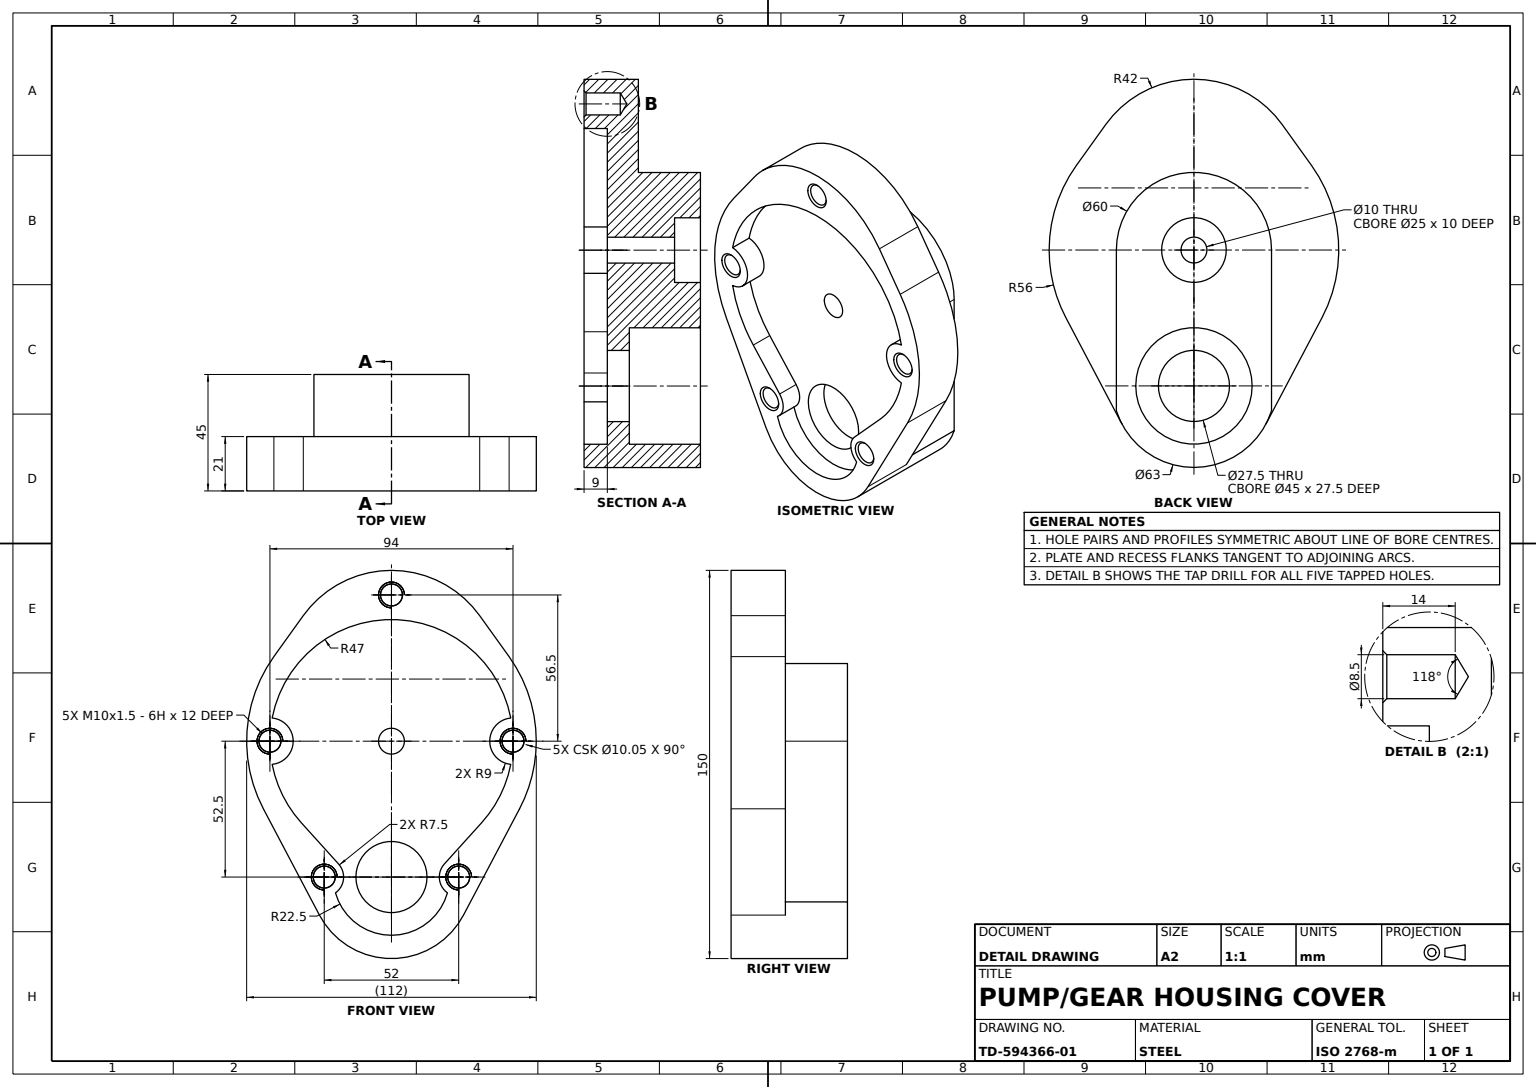
solid
v1 (0,48.5,34.11378)
v2 (21,48.5,34.11378)
e1 v1 v2 LINE
v3 (21,48.5,-34.11378)
e2 v3 v2 CIRCLE(AX(P(21,24,0),D(1,0,0),D(0,0,-1)),42)
v4 (0,48.5,-34.11378)
e3 v4 v3 LINE
e4 v4 v1 CIRCLE(AX(P(0,24,0),D(1,0,0),D(0,0,-1)),42)
face CYL(AX(P(0,24,0),D(1,0,0),D(0,0,-1)),42) [e1 -e2 -e3 e4]
v5 (20.225,0,42.75)
v6 (21,0,41.975)
e5 v5 v6 LINE
v7 (20.225,0,51.25)
e6 v7 v5 CIRCLE(AX(P(20.225,0,47),D(1,0,0),D(0,0,-1)),4.25)
v8 (21,0,52.025)
e7 v7 v8 LINE
e8 v8 v6 CIRCLE(AX(P(21,0,47),D(1,0,0),D(0,0,-1)),5.025)
face CONE(AX(P(21,0,47),D(1,0,0),D(0,0,-1)),5.025,0.785398163) rev [-e5 -e6 e7 e8]
v9 (12,-31.528256,-34.856407)
v10 (21,-31.528256,-34.856407)
e9 v9 v10 LINE
v11 (12,-47.468895,-20.437807)
e10 v11 v9 LINE
v12 (21,-47.468895,-20.437807)
e11 v11 v12 LINE
e12 v12 v10 LINE
face PLANE(AX(P(12,-47.468895,-20.437807),D(0,-0.670813951,-0.741625676),D(0,0.741625676,-0.670813951))) rev [-e9 -e10 e11 e12]
v13 (7,-52.5,30.25)
v14 (7,-52.5,21.75)
e13 v13 v14 CIRCLE(AX(P(7,-52.5,26),D(1,0,0),D(0,0,-1)),4.25)
v15 (4.446342,-52.5,26)
e14 v15 v14 LINE
e15 v15 v13 LINE
face CONE(AX(P(7,-52.5,26),D(1,0,0),D(0,0,-1)),4.25,1.029744259) rev [e13 -e14 e15]
v16 (12,-52.5,13.75)
v17 (3.5,-52.5,13.75)
e16 v16 v17 LINE
v18 (12,-52.5,-13.75)
e17 v16 v18 CIRCLE(AX(P(12,-52.5,0),D(1,0,0),D(0,0,-1)),13.75)
v19 (3.5,-52.5,-13.75)
e18 v18 v19 LINE
e19 v19 v17 CIRCLE(AX(P(3.5,-52.5,0),D(-1,0,0),D(0,0,1)),13.75)
face CYL(AX(P(-24,-52.5,0),D(-1,0,0),D(0,0,1)),13.75) rev [-e16 e17 e18 e19]
v20 (7,0,42.75)
v21 (7,0,51.25)
e20 v20 v21 CIRCLE(AX(P(7,0,47),D(1,0,0),D(0,0,-1)),4.25)
v22 (4.446342,0,47)
e21 v22 v21 LINE
e22 v22 v20 LINE
face CONE(AX(P(7,0,47),D(1,0,0),D(0,0,-1)),4.25,1.029744259) rev [e20 -e21 e22]
v23 (12,-47.468895,20.437807)
v24 (21,-47.468895,20.437807)
e23 v23 v24 LINE
v25 (12,-31.528256,34.856407)
e24 v25 v23 LINE
v26 (21,-31.528256,34.856407)
e25 v25 v26 LINE
e26 v26 v24 LINE
face PLANE(AX(P(12,-47.468895,20.437807),D(0,-0.670813951,0.741625676),D(0,-0.741625676,-0.670813951))) rev [-e23 -e24 e25 e26]
v27 (-24,0,12.5)
v28 (-24,0,-12.5)
e27 v27 v28 CIRCLE(AX(P(-24,0,0),D(-1,0,0),D(0,0,1)),12.5)
v29 (-14,0,-12.5)
e28 v29 v28 LINE
v30 (-14,0,12.5)
e29 v30 v29 CIRCLE(AX(P(-14,0,0),D(-1,0,0),D(0,0,1)),12.5)
e30 v30 v27 LINE
face CYL(AX(P(-24,0,0),D(-1,0,0),D(0,0,1)),12.5) rev [e27 -e28 -e29 e30]
v31 (0,32.666667,45.48504)
e31 v1 v31 LINE
v32 (21,32.666667,45.48504)
e32 v31 v32 LINE
e33 v2 v32 LINE
face PLANE(AX(P(0,32.666667,45.48504),D(0,0.583333333,0.812232862),D(0,-0.812232862,0.583333333))) [-e1 e31 e32 -e33]
v33 (-24,-62.104686,-30)
v34 (0,-62.104686,-30)
e34 v33 v34 LINE
v35 (-24,0,-30)
e35 v35 v33 LINE
v36 (0,0,-30)
e36 v35 v36 LINE
e37 v36 v34 LINE
face PLANE(AX(P(-24,0,-30),D(0,0,1),D(0,-1,0))) rev [-e34 -e35 e36 e37]
v37 (4.446342,0,-47)
v38 (7,0,-51.25)
e38 v37 v38 LINE
v39 (7,0,-42.75)
e39 v37 v39 LINE
e40 v39 v38 CIRCLE(AX(P(7,0,-47),D(1,0,0),D(0,0,-1)),4.25)
face CONE(AX(P(7,0,-47),D(1,0,0),D(0,0,-1)),4.25,1.029744259) rev [-e38 e39 e40]
v40 (0,-26.133333,-49.528264)
v41 (0,0,-56)
e41 v40 v41 CIRCLE(AX(P(0,0,0),D(1,0,0),D(0,0,-1)),56)
v42 (21,0,-56)
e42 v41 v42 LINE
v43 (21,-26.133333,-49.528264)
e43 v43 v42 CIRCLE(AX(P(21,0,0),D(1,0,0),D(0,0,-1)),56)
e44 v40 v43 LINE
face CYL(AX(P(0,0,0),D(1,0,0),D(0,0,-1)),56) [e41 e42 -e43 -e44]
v44 (20.225,-52.5,-21.75)
v45 (21,-52.5,-20.975)
e45 v44 v45 LINE
v46 (20.225,-52.5,-30.25)
e46 v46 v44 CIRCLE(AX(P(20.225,-52.5,-26),D(1,0,0),D(0,0,-1)),4.25)
v47 (21,-52.5,-31.025)
e47 v46 v47 LINE
e48 v47 v45 CIRCLE(AX(P(21,-52.5,-26),D(1,0,0),D(0,0,-1)),5.025)
face CONE(AX(P(21,-52.5,-26),D(1,0,0),D(0,0,-1)),5.025,0.785398163) rev [-e45 -e46 e47 e48]
e49 v21 v20 CIRCLE(AX(P(7,0,47),D(1,0,0),D(0,0,-1)),4.25)
face CONE(AX(P(7,0,47),D(1,0,0),D(0,0,-1)),4.25,1.029744259) rev [e21 e49 -e22]
v48 (20.225,-52.5,30.25)
e50 v13 v48 LINE
e51 v14 v13 CIRCLE(AX(P(7,-52.5,26),D(1,0,0),D(0,0,-1)),4.25)
v49 (20.225,-52.5,21.75)
e52 v14 v49 LINE
e53 v49 v48 CIRCLE(AX(P(20.225,-52.5,26),D(1,0,0),D(0,0,-1)),4.25)
face CYL(AX(P(21,-52.5,26),D(1,0,0),D(0,0,-1)),4.25) rev [-e50 -e51 e52 e53]
v50 (7,56.5,-4.25)
v51 (20.225,56.5,-4.25)
e54 v50 v51 LINE
v52 (20.225,56.5,4.25)
e55 v51 v52 CIRCLE(AX(P(20.225,56.5,0),D(1,0,0),D(0,0,-1)),4.25)
v53 (7,56.5,4.25)
e56 v53 v52 LINE
e57 v50 v53 CIRCLE(AX(P(7,56.5,0),D(1,0,0),D(0,0,-1)),4.25)
face CYL(AX(P(21,56.5,0),D(1,0,0),D(0,0,-1)),4.25) rev [e54 e55 -e56 -e57]
v54 (21,-26.133333,49.528264)
v55 (21,-67.2,27.859648)
e58 v54 v55 LINE
v56 (0,-26.133333,49.528264)
e59 v56 v54 LINE
v57 (0,-67.2,27.859648)
e60 v56 v57 LINE
e61 v57 v55 LINE
face PLANE(AX(P(0,-26.133333,49.528264),D(0,-0.466666667,0.884433277),D(0,-0.884433277,-0.466666667))) [-e58 -e59 e60 e61]
v58 (4.446342,56.5,0)
e62 v58 v53 LINE
e63 v58 v50 LINE
face CONE(AX(P(7,56.5,0),D(1,0,0),D(0,0,-1)),4.25,1.029744259) rev [-e62 e63 e57]
v59 (4.446342,-52.5,-26)
v60 (7,-52.5,-30.25)
e64 v59 v60 LINE
v61 (7,-52.5,-21.75)
e65 v60 v61 CIRCLE(AX(P(7,-52.5,-26),D(1,0,0),D(0,0,-1)),4.25)
e66 v59 v61 LINE
face CONE(AX(P(7,-52.5,-26),D(1,0,0),D(0,0,-1)),4.25,1.029744259) rev [e64 e65 -e66]
v62 (12,-8.958653,-46.138298)
v63 (21,-8.958653,-46.138298)
e67 v62 v63 LINE
v64 (21,8.958653,-46.138298)
e68 v63 v64 CIRCLE(AX(P(21,0,-47),D(-1,0,0),D(0,0,1)),9)
v65 (12,8.958653,-46.138298)
e69 v65 v64 LINE
e70 v62 v65 CIRCLE(AX(P(12,0,-47),D(-1,0,0),D(0,0,1)),9)
face CYL(AX(P(12,0,-47),D(1,0,0),D(0,0,-1)),9) [e67 e68 -e69 -e70]
v66 (12,8.958653,46.138298)
v67 (12,0,38)
e71 v66 v67 CIRCLE(AX(P(12,0,47),D(-1,0,0),D(0,0,-1)),9)
v68 (12,-8.958653,46.138298)
e72 v67 v68 CIRCLE(AX(P(12,0,47),D(-1,0,0),D(0,0,-1)),9)
e73 v68 v25 CIRCLE(AX(P(12,0,0),D(1,0,0),D(0,0,-1)),47)
v69 (12,-52.5,18.5)
e74 v23 v69 CIRCLE(AX(P(12,-52.5,26),D(-1,0,0),D(0,0,1)),7.5)
v70 (12,-58.61236,21.653846)
e75 v69 v70 CIRCLE(AX(P(12,-52.5,26),D(-1,0,0),D(0,0,1)),7.5)
v71 (12,-58.61236,-21.653846)
e76 v70 v71 CIRCLE(AX(P(12,-52.5,0),D(1,0,0),D(0,0,-1)),22.5)
e77 v71 v11 CIRCLE(AX(P(12,-52.5,-26),D(-1,0,0),D(0,0,-1)),7.5)
e78 v9 v62 CIRCLE(AX(P(12,0,0),D(1,0,0),D(0,0,-1)),47)
e79 v65 v66 CIRCLE(AX(P(12,0,0),D(1,0,0),D(0,0,-1)),47)
e80 v18 v16 CIRCLE(AX(P(12,-52.5,0),D(1,0,0),D(0,0,-1)),13.75)
v72 (12,0,5)
v73 (12,0,-5)
e81 v72 v73 CIRCLE(AX(P(12,0,0),D(1,0,0),D(0,0,-1)),5)
e82 v73 v72 CIRCLE(AX(P(12,0,0),D(1,0,0),D(0,0,-1)),5)
face PLANE(AX(P(12,0,0),D(1,0,0),D(0,0,-1))) [e71 e72 e73 e24 e74 e75 e76 e77 e10 e78 e70 e79] [-e17 -e80] [-e81 -e82]
e83 v48 v49 CIRCLE(AX(P(20.225,-52.5,26),D(1,0,0),D(0,0,-1)),4.25)
face CYL(AX(P(21,-52.5,26),D(1,0,0),D(0,0,-1)),4.25) rev [e50 e83 -e52 -e13]
v74 (-24,-62.104686,30)
v75 (-24,0,30)
e84 v74 v75 LINE
v76 (0,-62.104686,30)
e85 v74 v76 LINE
v77 (0,0,30)
e86 v76 v77 LINE
e87 v75 v77 LINE
face PLANE(AX(P(-24,0,30),D(0,0,-1),D(0,1,0))) rev [-e84 e85 e86 -e87]
e88 v17 v19 CIRCLE(AX(P(3.5,-52.5,0),D(-1,0,0),D(0,0,1)),13.75)
face CYL(AX(P(-24,-52.5,0),D(-1,0,0),D(0,0,1)),13.75) rev [e16 e88 -e18 e80]
v78 (21,56.5,-5.025)
e89 v51 v78 LINE
v79 (21,56.5,5.025)
e90 v78 v79 CIRCLE(AX(P(21,56.5,0),D(1,0,0),D(0,0,-1)),5.025)
e91 v52 v79 LINE
face CONE(AX(P(21,56.5,0),D(1,0,0),D(0,0,-1)),5.025,0.785398163) rev [e89 e90 -e91 -e55]
v80 (21,8.958653,46.138298)
e92 v64 v80 CIRCLE(AX(P(21,0,0),D(1,0,0),D(0,0,-1)),47)
e93 v66 v80 LINE
face CYL(AX(P(12,0,0),D(1,0,0),D(0,0,-1)),47) rev [-e79 e69 e92 -e93]
e94 v61 v60 CIRCLE(AX(P(7,-52.5,-26),D(1,0,0),D(0,0,-1)),4.25)
e95 v61 v44 LINE
e96 v44 v46 CIRCLE(AX(P(20.225,-52.5,-26),D(1,0,0),D(0,0,-1)),4.25)
e97 v60 v46 LINE
face CYL(AX(P(21,-52.5,-26),D(1,0,0),D(0,0,-1)),4.25) rev [-e94 e95 e96 -e97]
e98 v38 v39 CIRCLE(AX(P(7,0,-47),D(1,0,0),D(0,0,-1)),4.25)
face CONE(AX(P(7,0,-47),D(1,0,0),D(0,0,-1)),4.25,1.029744259) rev [e98 -e39 e38]
face CONE(AX(P(7,-52.5,26),D(1,0,0),D(0,0,-1)),4.25,1.029744259) rev [e51 -e15 e14]
face CONE(AX(P(7,-52.5,-26),D(1,0,0),D(0,0,-1)),4.25,1.029744259) rev [e94 -e64 e66]
v81 (21,-52.5,20.975)
e99 v49 v81 LINE
v82 (21,-52.5,31.025)
e100 v81 v82 CIRCLE(AX(P(21,-52.5,26),D(1,0,0),D(0,0,-1)),5.025)
e101 v48 v82 LINE
face CONE(AX(P(21,-52.5,26),D(1,0,0),D(0,0,-1)),5.025,0.785398163) rev [-e53 e99 e100 -e101]
face CYL(AX(P(21,-52.5,-26),D(1,0,0),D(0,0,-1)),4.25) rev [e97 e46 -e95 -e65]
v83 (-24,-52.5,-22.5)
v84 (-24,-52.5,22.5)
e102 v83 v84 CIRCLE(AX(P(-24,-52.5,0),D(-1,0,0),D(0,0,1)),22.5)
v85 (3.5,-52.5,22.5)
e103 v85 v84 LINE
v86 (3.5,-52.5,-22.5)
e104 v86 v85 CIRCLE(AX(P(3.5,-52.5,0),D(-1,0,0),D(0,0,1)),22.5)
e105 v86 v83 LINE
face CYL(AX(P(-24,-52.5,0),D(-1,0,0),D(0,0,1)),22.5) rev [e102 -e103 -e104 e105]
e106 v82 v81 CIRCLE(AX(P(21,-52.5,26),D(1,0,0),D(0,0,-1)),5.025)
face CONE(AX(P(21,-52.5,26),D(1,0,0),D(0,0,-1)),5.025,0.785398163) rev [-e83 e101 e106 -e99]
v87 (-14,0,5)
v88 (-14,0,-5)
e107 v87 v88 CIRCLE(AX(P(-14,0,0),D(-1,0,0),D(0,0,1)),5)
e108 v73 v88 LINE
e109 v72 v87 LINE
face CYL(AX(P(-24,0,0),D(-1,0,0),D(0,0,1)),5) rev [e107 -e108 e82 e109]
e110 v21 v7 LINE
e111 v20 v5 LINE
face CYL(AX(P(21,0,47),D(1,0,0),D(0,0,-1)),4.25) rev [-e49 e110 e6 -e111]
e112 v88 v87 CIRCLE(AX(P(-14,0,0),D(-1,0,0),D(0,0,1)),5)
face CYL(AX(P(-24,0,0),D(-1,0,0),D(0,0,1)),5) rev [e81 e108 e112 -e109]
v89 (21,0,38)
v90 (21,-8.958653,46.138298)
e113 v89 v90 CIRCLE(AX(P(21,0,47),D(-1,0,0),D(0,0,-1)),9)
e114 v68 v90 LINE
e115 v67 v89 LINE
face CYL(AX(P(12,0,47),D(1,0,0),D(0,0,-1)),9) [e113 -e114 -e72 e115]
v91 (21,0,-41.975)
v92 (21,0,-52.025)
e116 v91 v92 CIRCLE(AX(P(21,0,-47),D(1,0,0),D(0,0,-1)),5.025)
e117 v92 v91 CIRCLE(AX(P(21,0,-47),D(1,0,0),D(0,0,-1)),5.025)
v93 (21,-67.2,-27.859648)
e118 v93 v43 LINE
v94 (21,32.666667,-45.48504)
e119 v42 v94 CIRCLE(AX(P(21,0,0),D(1,0,0),D(0,0,-1)),56)
e120 v94 v3 LINE
e121 v32 v54 CIRCLE(AX(P(21,0,0),D(1,0,0),D(0,0,-1)),56)
e122 v55 v93 CIRCLE(AX(P(21,-52.5,0),D(1,0,0),D(0,0,-1)),31.5)
e123 v45 v47 CIRCLE(AX(P(21,-52.5,-26),D(1,0,0),D(0,0,-1)),5.025)
e124 v79 v78 CIRCLE(AX(P(21,56.5,0),D(1,0,0),D(0,0,-1)),5.025)
e125 v80 v89 CIRCLE(AX(P(21,0,47),D(-1,0,0),D(0,0,-1)),9)
e126 v10 v63 CIRCLE(AX(P(21,0,0),D(1,0,0),D(0,0,-1)),47)
v95 (21,-58.61236,-21.653846)
e127 v95 v12 CIRCLE(AX(P(21,-52.5,-26),D(-1,0,0),D(0,0,-1)),7.5)
v96 (21,-58.61236,21.653846)
e128 v96 v95 CIRCLE(AX(P(21,-52.5,0),D(1,0,0),D(0,0,-1)),22.5)
v97 (21,-52.5,18.5)
e129 v97 v96 CIRCLE(AX(P(21,-52.5,26),D(-1,0,0),D(0,0,1)),7.5)
e130 v24 v97 CIRCLE(AX(P(21,-52.5,26),D(-1,0,0),D(0,0,1)),7.5)
e131 v90 v26 CIRCLE(AX(P(21,0,0),D(1,0,0),D(0,0,-1)),47)
e132 v6 v8 CIRCLE(AX(P(21,0,47),D(1,0,0),D(0,0,-1)),5.025)
face PLANE(AX(P(21,0,0),D(1,0,0),D(0,0,-1))) [-e116 -e117] [e118 e43 e119 e120 e2 e33 e121 e58 e122] [-e48 -e123] [-e106 -e100] [-e124 -e90] [-e125 -e92 -e68 -e126 -e12 -e127 -e128 -e129 -e130 -e26 -e131 -e113] [-e8 -e132]
e133 v70 v96 LINE
e134 v71 v95 LINE
face CYL(AX(P(12,-52.5,0),D(1,0,0),D(0,0,-1)),22.5) rev [e133 e128 -e134 -e76]
face CONE(AX(P(21,-52.5,-26),D(1,0,0),D(0,0,-1)),5.025,0.785398163) rev [-e47 -e96 e45 e123]
e135 v69 v97 LINE
face CYL(AX(P(12,-52.5,26),D(1,0,0),D(0,0,-1)),7.5) [e130 -e135 -e74 e23]
e136 v29 v30 CIRCLE(AX(P(-14,0,0),D(-1,0,0),D(0,0,1)),12.5)
face PLANE(AX(P(-14,5,0),D(1,0,0),D(0,0,-1))) rev [e136 e29] [-e112 -e107]
face CYL(AX(P(12,-52.5,-26),D(1,0,0),D(0,0,-1)),7.5) [e127 -e11 -e77 e134]
e137 v53 v50 CIRCLE(AX(P(7,56.5,0),D(1,0,0),D(0,0,-1)),4.25)
face CONE(AX(P(7,56.5,0),D(1,0,0),D(0,0,-1)),4.25,1.029744259) rev [-e63 e62 e137]
v98 (0,32.666667,-45.48504)
e138 v41 v98 CIRCLE(AX(P(0,0,0),D(1,0,0),D(0,0,-1)),56)
e139 v98 v94 LINE
face CYL(AX(P(0,0,0),D(1,0,0),D(0,0,-1)),56) [-e119 -e42 e138 e139]
face CYL(AX(P(12,0,47),D(1,0,0),D(0,0,-1)),9) [-e115 -e71 e93 e125]
face CYL(AX(P(12,0,0),D(1,0,0),D(0,0,-1)),47) rev [e9 e126 -e67 -e78]
e140 v98 v4 LINE
face PLANE(AX(P(0,32.666667,-45.48504),D(0,0.583333333,-0.812232862),D(0,0.812232862,0.583333333))) [-e120 -e139 e140 e3]
e141 v31 v56 CIRCLE(AX(P(0,0,0),D(1,0,0),D(0,0,-1)),56)
face CYL(AX(P(0,0,0),D(1,0,0),D(0,0,-1)),56) [-e121 -e32 e141 e59]
v99 (20.225,0,-42.75)
v100 (20.225,0,-51.25)
e142 v99 v100 CIRCLE(AX(P(20.225,0,-47),D(1,0,0),D(0,0,-1)),4.25)
e143 v38 v100 LINE
e144 v39 v99 LINE
face CYL(AX(P(21,0,-47),D(1,0,0),D(0,0,-1)),4.25) rev [e142 -e143 -e40 e144]
e145 v100 v99 CIRCLE(AX(P(20.225,0,-47),D(1,0,0),D(0,0,-1)),4.25)
face CYL(AX(P(21,0,-47),D(1,0,0),D(0,0,-1)),4.25) rev [e145 -e144 -e98 e143]
e146 v52 v51 CIRCLE(AX(P(20.225,56.5,0),D(1,0,0),D(0,0,-1)),4.25)
face CYL(AX(P(21,56.5,0),D(1,0,0),D(0,0,-1)),4.25) rev [e56 e146 -e54 -e137]
e147 v5 v7 CIRCLE(AX(P(20.225,0,47),D(1,0,0),D(0,0,-1)),4.25)
face CYL(AX(P(21,0,47),D(1,0,0),D(0,0,-1)),4.25) rev [e111 e147 -e110 -e20]
e148 v85 v86 CIRCLE(AX(P(3.5,-52.5,0),D(-1,0,0),D(0,0,1)),22.5)
face PLANE(AX(P(3.5,-38.75,0),D(1,0,0),D(0,0,-1))) rev [e148 e104] [-e88 -e19]
face CONE(AX(P(21,56.5,0),D(1,0,0),D(0,0,-1)),5.025,0.785398163) rev [-e146 e91 e124 -e89]
v101 (0,-67.2,-27.859648)
e149 v101 v93 LINE
e150 v101 v40 LINE
face PLANE(AX(P(0,-26.133333,-49.528264),D(0,-0.466666667,-0.884433277),D(0,0.884433277,-0.466666667))) [-e118 -e149 e150 e44]
e151 v75 v35 CIRCLE(AX(P(-24,0,0),D(-1,0,0),D(0,0,1)),30)
e152 v77 v36 CIRCLE(AX(P(0,0,0),D(-1,0,0),D(0,0,1)),30)
face CYL(AX(P(-24,0,0),D(1,0,0),D(0,0,-1)),30) [-e151 e87 e152 -e36]
e153 v100 v92 LINE
e154 v99 v91 LINE
face CONE(AX(P(21,0,-47),D(1,0,0),D(0,0,-1)),5.025,0.785398163) rev [e116 -e153 -e142 e154]
face CYL(AX(P(12,-52.5,26),D(1,0,0),D(0,0,-1)),7.5) [e135 e129 -e133 -e75]
face CYL(AX(P(12,0,0),D(1,0,0),D(0,0,-1)),47) rev [-e25 -e73 e114 e131]
e155 v33 v74 CIRCLE(AX(P(-24,-52.5,0),D(-1,0,0),D(0,0,1)),31.5)
e156 v28 v27 CIRCLE(AX(P(-24,0,0),D(-1,0,0),D(0,0,1)),12.5)
e157 v84 v83 CIRCLE(AX(P(-24,-52.5,0),D(-1,0,0),D(0,0,1)),22.5)
face PLANE(AX(P(-24,0,0),D(-1,0,0),D(0,0,1))) [e151 e35 e155 e84] [-e156 -e27] [-e102 -e157]
face CONE(AX(P(21,0,47),D(1,0,0),D(0,0,-1)),5.025,0.785398163) rev [e5 e132 -e7 -e147]
e158 v34 v101 CIRCLE(AX(P(0,-52.5,0),D(-1,0,0),D(0,0,1)),31.5)
e159 v57 v76 CIRCLE(AX(P(0,-52.5,0),D(-1,0,0),D(0,0,1)),31.5)
face PLANE(AX(P(0,0,0),D(1,0,0),D(0,0,-1))) rev [-e60 -e141 -e31 -e4 -e140 -e138 -e41 -e150 -e158 -e37 -e152 -e86 -e159]
face CYL(AX(P(-24,0,0),D(-1,0,0),D(0,0,1)),12.5) rev [-e136 e28 e156 -e30]
face CYL(AX(P(0,-52.5,0),D(1,0,0),D(0,0,-1)),31.5) [e158 e149 -e122 -e61 e159 -e85 -e155 e34]
face CYL(AX(P(-24,-52.5,0),D(-1,0,0),D(0,0,1)),22.5) rev [-e105 -e148 e103 e157]
face CONE(AX(P(21,0,-47),D(1,0,0),D(0,0,-1)),5.025,0.785398163) rev [-e154 -e145 e153 e117]
